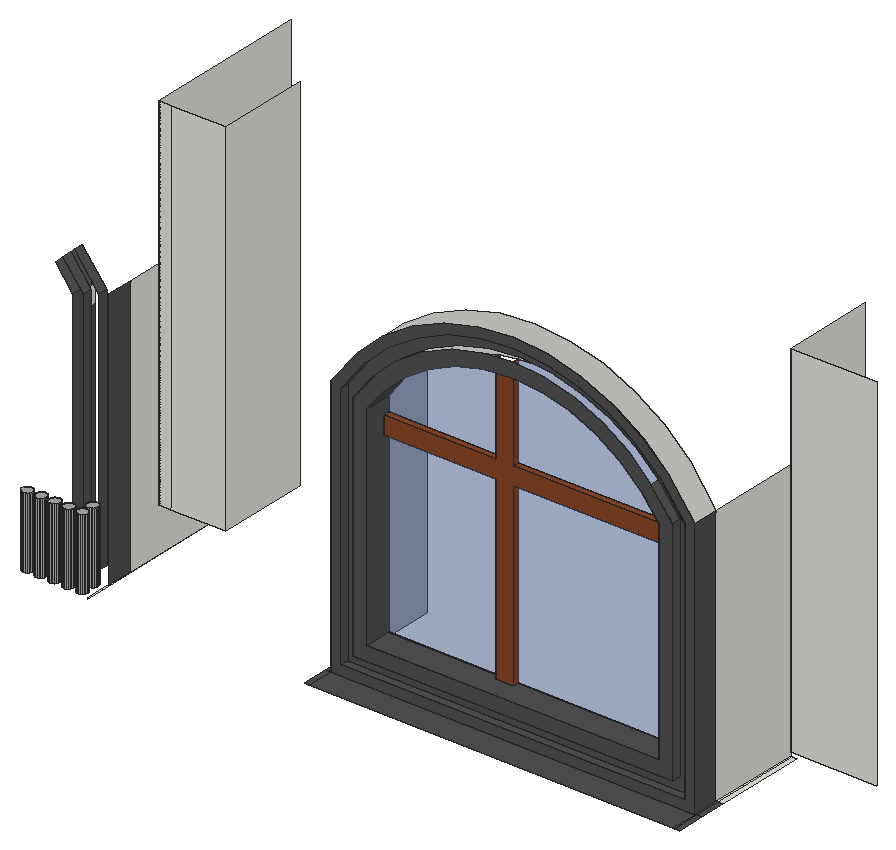
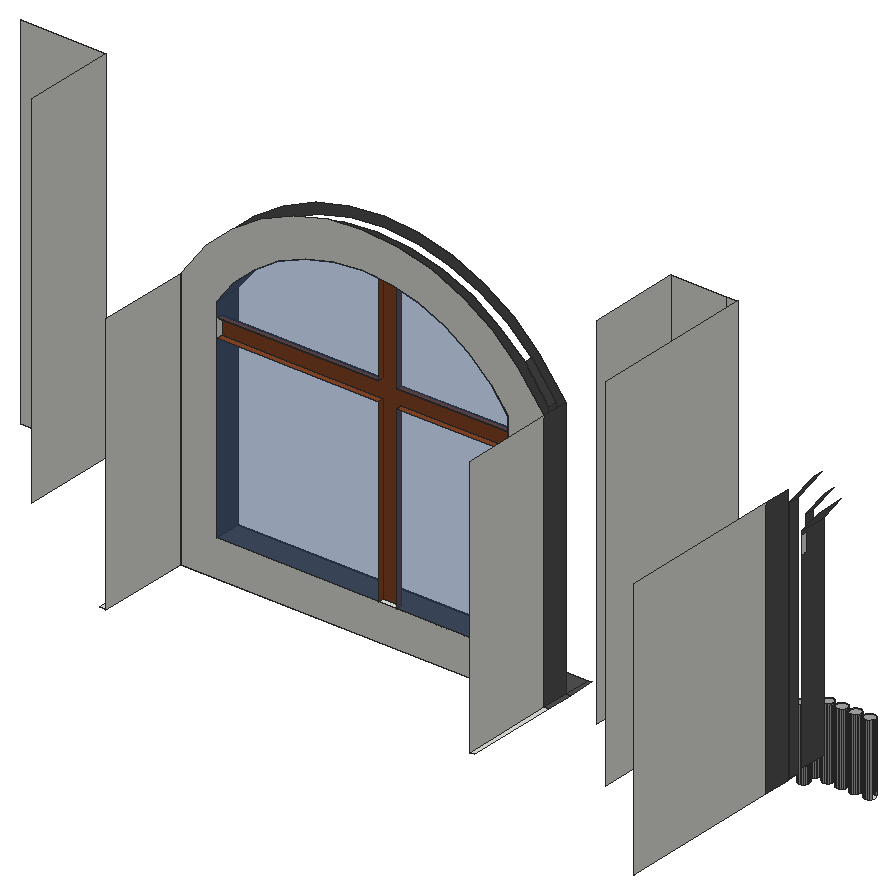
# SketchUp Ruby script. Lengths in inches.
U = 1.inch
M = Sketchup.active_model
def pt(a) = Geom::Point3d.new(a.map { |v| v * U })
def face(e, loops, mat)
  f = e.add_face(loops[0].map { |a| pt(a) })
  loops[1..].each { |l| e.add_face(l.map { |a| pt(a) }).erase! }
  f.material = f.back_material = mat if mat
  f
end
# faces: each face lists its corners as indices into pts; further lists are holes
def faces(e, pts, list, mat = nil) = list.each { |f| face(e, (f[0].is_a?(Array) ? f : [f]).map { |l| l.map { |i| pts[i] } }, mat) }
# xy, xz, yz: faces in a plane at the given z, y or x. An outline is a flat list of corners, or four numbers for a rectangle; further outlines are holes
def ring(l) = l.size == 4 ? [[l[0], l[1]], [l[2], l[1]], [l[2], l[3]], [l[0], l[3]]] : l.each_slice(2).to_a
def flat(e, list, mat, &to3) = list.each { |f| face(e, (f[0].is_a?(Array) ? f : [f]).map { |l| ring(l).map { |u, v| to3.(u, v) } }, mat) }
def xy(e, z, list, mat = nil) = flat(e, list, mat) { |x, y| [x, y, z] }
def xz(e, y, list, mat = nil) = flat(e, list, mat) { |x, z| [x, y, z] }
def yz(e, x, list, mat = nil) = flat(e, list, mat) { |y, z| [x, y, z] }
def lines(e, pts, list) = list.each { |a, b| e.add_line(pt(pts[a]), pt(pts[b])) }
# prism: a flat outline (further loops are holes) pulled along v
def prism(e, loops, v, mat = nil)
  f = face(e, loops, mat); d = Geom::Vector3d.new(v.map { |x| x * U })
  f.pushpull(f.normal.samedirection?(d) ? d.length : -d.length)
end
def box(e, o, s, mat = nil) = prism(e, [[o, [o[0] + s[0], o[1], o[2]], [o[0] + s[0], o[1] + s[1], o[2]], [o[0], o[1] + s[1], o[2]]]], [0, 0, s[2]], mat)
def at(x, y, z, deg = 0) = Geom::Transformation.translation(pt([x, y, z])) * Geom::Transformation.rotation(ORIGIN, Z_AXIS, deg.degrees)
def axes(o, x, y, z) = Geom::Transformation.new([*x, 0, *y, 0, *z, 0, *pt(o).to_a, 1])
def part(name) = M.definitions.add(name)
# library, detail: a bought-in or finely detailed component or shape, given as its bounding box
def library(name, o, s) = part(name).tap { |d| box(d.entities, o, s) }
def detail(e, o, s) = box(e.add_group.entities, o, s)
def put(e, d, t, mat = nil) = e.add_instance(d, t).tap { |i| i.material = mat if mat }
def group(e, t, mat = nil) = e.add_group.tap { |g| g.transformation = t; g.material = mat if mat }.entities
root = M.entities
M.materials.add("[0042_Sienna]").color = [137, 70, 38]
M.materials.add("[0132_LightGray]").color = [169, 169, 169]
M.materials.add("[0135_DarkGray]").color = [81, 81, 81]
M.materials.add("[Translucent Glass Blue]").color = [66, 99, 158]
M.materials["[Translucent Glass Blue]"].alpha = 0.5
xy(root,336.85,[[361.14,31.6875,361.32,37.6875],[339.27,32.1,338.81,32.2,338.39,32.42,338.04,32.73,337.78,33.13,337.63,33.58,337.61,34.05,337.7,34.52,337.92,34.9375,338.23,35.29,338.63,35.55,339.08,35.69,339.55,35.72,340.02,35.62,340.4375,35.41,340.79,35.09,341.05,34.69,341.19,34.24,341.22,33.77,341.12,33.31,340.91,32.89,340.59,32.53,340.19,32.28,339.74,32.13],[343.83,32.1,343.37,32.2,342.95,32.42,342.6,32.73,342.34,33.13,342.19,33.58,342.17,34.05,342.27,34.52,342.48,34.9375,342.8,35.29,343.19,35.55,343.64,35.69,344.12,35.72,344.58,35.62,345,35.41,345.35,35.09,345.61,34.69,345.76,34.24,345.78,33.77,345.68,33.31,345.47,32.89,345.15,32.53,344.76,32.28,344.31,32.13],[348.4,32.1,347.93,32.2,347.51,32.42,347.16,32.73,346.9,33.13,346.76,33.58,346.73,34.05,346.83,34.52,347.04,34.9375,347.36,35.29,347.76,35.55,348.21,35.69,348.68,35.72,349.14,35.62,349.5625,35.41,349.92,35.09,350.17,34.69,350.32,34.24,350.34,33.77,350.25,33.31,350.03,32.89,349.72,32.53,349.32,32.28,348.87,32.13],[352.96,32.1,352.5,32.2,352.07,32.42,351.72,32.73,351.47,33.13,351.32,33.58,351.29,34.05,351.39,34.52,351.61,34.9375,351.92,35.29,352.32,35.55,352.77,35.69,353.24,35.72,353.7,35.62,354.125,35.41,354.48,35.09,354.74,34.69,354.88,34.24,354.91,33.77,354.81,33.31,354.59,32.89,354.28,32.53,353.88,32.28,353.43,32.13],
  [357.52,32.1,357.06,32.2,356.64,32.42,356.29,32.73,356.03,33.13,355.88,33.58,355.86,34.05,355.95,34.52,356.17,34.9375,356.48,35.29,356.88,35.55,357.33,35.69,357.8,35.72,358.27,35.62,358.6875,35.41,359.04,35.09,359.3,34.69,359.44,34.24,359.47,33.77,359.37,33.31,359.16,32.89,358.84,32.53,358.44,32.28,357.99,32.13],[361.14,37.6875,361.32,49.6875],[434.7,40.6875,555.39,49.6875],[361.14,49.6875,361.32,104.375],[433.14,49.6875,434.7,80.4375],
  [555.39,49.6875,556.01,80.4375],[556.01,49.6875,557.64,80.4375]])
xy(root,336.85,[[433.14,31.6875,434.7,40.6875],[434.7,31.6875,555.39,40.6875],[555.39,31.6875,556.01,40.6875],[556.01,31.6875,557.64,40.6875],[433.14,40.6875,434.7,49.6875],
  [555.39,40.6875,556.01,49.6875],[556.01,40.6875,557.64,49.6875]],"[0135_DarkGray]")
xy(root,340.02,[[437.88,40.6875,552.21,43.6875]],"[0135_DarkGray]")
xy(root,344.17,[[442.02,40.6875,548.06,43.6875]],"[0135_DarkGray]")
xy(root,348.85,[[483.7,47.6875,489.7,49.6875]])
xy(root,348.85,[[446.7,40.6875,543.39,40.6875,543.39,49.6875,489.7,49.6875,489.7,47.6875,483.7,47.6875,483.7,49.6875,446.7,49.6875]],"[0135_DarkGray]")
xy(root,360.41,[[339.27,32.1,339.74,32.13,340.19,32.28,340.59,32.53,340.91,32.89,341.12,33.31,341.22,33.77,341.19,34.24,341.05,34.69,340.79,35.09,340.4375,35.41,340.02,35.62,339.55,35.72,339.08,35.69,338.63,35.55,338.23,35.29,337.92,34.9375,337.7,34.52,337.61,34.05,337.63,33.58,337.78,33.13,338.04,32.73,338.39,32.42,338.81,32.2],[343.83,32.1,344.31,32.13,344.76,32.28,345.15,32.53,345.47,32.89,345.68,33.31,345.78,33.77,345.76,34.24,345.61,34.69,345.35,35.09,345,35.41,344.58,35.62,344.12,35.72,343.64,35.69,343.19,35.55,342.8,35.29,342.48,34.9375,342.27,34.52,342.17,34.05,342.19,33.58,342.34,33.13,342.6,32.73,342.95,32.42,343.37,32.2],[348.4,32.1,348.87,32.13,349.32,32.28,349.72,32.53,350.03,32.89,350.25,33.31,350.34,33.77,350.32,34.24,350.17,34.69,349.92,35.09,349.5625,35.41,349.14,35.62,348.68,35.72,348.21,35.69,347.76,35.55,347.36,35.29,347.04,34.9375,346.83,34.52,346.73,34.05,346.76,33.58,346.9,33.13,347.16,32.73,347.51,32.42,347.93,32.2],[352.96,32.1,353.43,32.13,353.88,32.28,354.28,32.53,354.59,32.89,354.81,33.31,354.91,33.77,354.88,34.24,354.74,34.69,354.48,35.09,354.125,35.41,353.7,35.62,353.24,35.72,352.77,35.69,352.32,35.55,351.92,35.29,351.61,34.9375,351.39,34.52,351.29,34.05,351.32,33.58,351.47,33.13,351.72,32.73,352.07,32.42,352.5,32.2],[357.52,32.1,357.99,32.13,358.44,32.28,358.84,32.53,359.16,32.89,359.37,33.31,359.47,33.77,359.44,34.24,359.3,34.69,359.04,35.09,358.6875,35.41,358.27,35.62,357.8,35.72,357.33,35.69,356.88,35.55,356.48,35.29,356.17,34.9375,355.95,34.52,355.86,34.05,355.88,33.58,356.03,33.13,356.29,32.73,356.64,32.42,357.06,32.2],
  [357.52,36.54,357.99,36.57,358.44,36.71,358.84,36.97,359.16,37.32,359.37,37.75,359.47,38.21,359.44,38.68,359.3,39.13,359.04,39.53,358.6875,39.84,358.27,40.06,357.8,40.16,357.33,40.13,356.88,39.98,356.48,39.73,356.17,39.375,355.95,38.95,355.86,38.49,355.88,38.02,356.03,37.57,356.29,37.17,356.64,36.85,357.06,36.64]],"[0132_LightGray]")
xy(root,408.35,[[446.7,47.6875,483.7,49.6875],[489.7,47.6875,543.39,49.6875]],"[0042_Sienna]")
xy(root,414.35,[[446.7,47.6875,483.7,49.6875],[489.7,47.6875,543.39,49.6875]],"[0042_Sienna]")
xz(root,40.6875,[[[434.7,336.85,555.39,336.85,555.39,423.26,546.46,434.86,537.99,442.73,528.34,449.09,517.76,453.76,506.5625,456.61,495.04,457.57,483.52,456.61,472.32,453.76,461.75,449.09,452.09,442.73,443.625,434.86,434.7,423.26],[437.88,340.02,437.88,422.18,445.98,432.71,454.0625,440.22,463.27,446.29,473.36,450.74,484.05,453.47,495.04,454.38,506.03,453.47,516.72,450.74,526.81,446.29,536.02,440.22,544.1,432.71,552.21,422.18,552.21,340.02]],[[442.02,344.17,548.06,344.17,548.06,420.77,541.02,429.91,533.45,436.95,524.82,442.63,515.36,446.81,505.34,449.36,495.04,450.22,484.74,449.36,474.72,446.81,465.27,442.63,456.63,436.95,449.06,429.91,442.02,420.77],[446.7,348.85,446.7,419.18,452.53,426.75,459.53,433.26,467.51,438.52,476.25,442.38,485.52,444.74,495.04,445.53,504.57,444.74,513.83,442.38,522.57,438.52,530.55,433.26,537.56,426.75,543.39,419.18,543.39,348.85]]],"[0135_DarkGray]")
xz(root,43.6875,[[[437.88,340.02,552.21,340.02,552.21,422.18,544.1,432.71,536.02,440.22,526.81,446.29,516.72,450.74,506.03,453.47,495.04,454.38,484.05,453.47,473.36,450.74,463.27,446.29,454.0625,440.22,445.98,432.71,437.88,422.18],[442.02,344.17,442.02,420.77,449.06,429.91,456.63,436.95,465.27,442.63,474.72,446.81,484.74,449.36,495.04,450.22,505.34,449.36,515.36,446.81,524.82,442.63,533.45,436.95,541.02,429.91,548.06,420.77,548.06,344.17]]],"[0135_DarkGray]")
xz(root,47.6875,[[483.7,348.85,489.7,348.85,489.7,408.35,543.39,408.35,543.39,414.35,489.7,414.35,489.7,445.09,485.52,444.74,483.7,444.27,483.7,414.35,446.7,414.35,446.7,408.35,483.7,408.35]],"[0042_Sienna]")
xz(root,49.6875,[[[434.7,336.85,434.7,423.26,443.625,434.86,452.09,442.73,461.75,449.09,472.32,453.76,483.52,456.61,495.04,457.57,506.5625,456.61,517.76,453.76,528.34,449.09,537.99,442.73,546.46,434.86,555.39,423.26,555.39,336.85],[446.7,348.85,543.39,348.85,543.39,419.18,537.56,426.75,530.55,433.26,522.57,438.52,513.83,442.38,504.57,444.74,495.04,445.53,489.7,445.09,485.52,444.74,483.7,444.27,476.25,442.38,467.51,438.52,459.53,433.26,452.53,426.75,446.7,419.18]],[370.55,360,370.74,480],[370.74,360,374.55,480],[374.55,360,392.7,480],[580.01,360,608.5,480]])
xz(root,49.6875,[[446.7,348.85,483.7,408.35],[489.7,348.85,543.39,408.35],[446.7,414.35,483.7,414.35,483.7,444.27,476.25,442.38,467.51,438.52,459.53,433.26,452.53,426.75,446.7,419.18],[489.7,414.35,543.39,414.35,543.39,419.18,537.56,426.75,530.55,433.26,522.57,438.52,513.83,442.38,504.57,444.74,495.04,445.53,489.7,445.09]],"[Translucent Glass Blue]")
yz(root,349.14,[[47.6875,412.18,49.6875,418.18]])
yz(root,349.14,[[40.6875,348.85,40.6875,419.18,49.6875,419.18,49.6875,418.18,47.6875,418.18,47.6875,412.18,49.6875,412.18,49.6875,348.85]],"[0135_DarkGray]")
yz(root,352.68,[[40.6875,345.3,43.6875,420.38]],"[0135_DarkGray]")
yz(root,357.84,[[40.6875,340.14,43.6875,422.14]],"[0135_DarkGray]")
yz(root,361.14,[[49.6875,336.85,104.375,423.26]])
yz(root,361.14,[[40.6875,336.85,49.6875,423.26]],"[0135_DarkGray]")
yz(root,370.55,[[49.6875,360,104.375,480]])
yz(root,392.7,[[49.6875,360,80.4375,480]])
yz(root,434.7,[[49.6875,336.85,80.4375,423.26]])
yz(root,434.7,[[40.6875,336.85,49.6875,423.26]],"[0135_DarkGray]")
yz(root,437.88,[[40.6875,340.02,43.6875,422.18]],"[0135_DarkGray]")
yz(root,442.02,[[40.6875,344.17,43.6875,420.77]],"[0135_DarkGray]")
yz(root,446.7,[[47.6875,408.35,49.6875,414.35]])
yz(root,446.7,[[40.6875,348.85,49.6875,348.85,49.6875,408.35,47.6875,408.35,47.6875,414.35,49.6875,414.35,49.6875,419.18,40.6875,419.18]],"[0135_DarkGray]")
yz(root,483.7,[[47.6875,348.85,49.6875,408.35],[47.6875,414.35,49.6875,444.27]],"[0042_Sienna]")
yz(root,489.7,[[47.6875,348.85,49.6875,408.35],[47.6875,414.35,49.6875,445.09]],"[0042_Sienna]")
yz(root,543.39,[[47.6875,408.35,49.6875,414.35]])
yz(root,543.39,[[40.6875,348.85,40.6875,419.18,49.6875,419.18,49.6875,414.35,47.6875,414.35,47.6875,408.35,49.6875,408.35,49.6875,348.85]],"[0135_DarkGray]")
yz(root,548.06,[[40.6875,344.17,43.6875,420.77]],"[0135_DarkGray]")
yz(root,552.21,[[40.6875,340.02,43.6875,422.18]],"[0135_DarkGray]")
yz(root,555.39,[[49.6875,336.85,80.4375,423.26]])
yz(root,555.39,[[40.6875,336.85,49.6875,423.26]],"[0135_DarkGray]")
yz(root,580.01,[[49.6875,360,80.4375,480]])
p = [[338.81,32.2,336.85],[339.27,32.1,336.85],[339.27,32.1,360.41],[338.81,32.2,360.41],[339.74,32.13,336.85],[339.74,32.13,360.41],
  [340.19,32.28,336.85],[340.19,32.28,360.41],[343.37,32.2,336.85],[343.83,32.1,336.85],[343.83,32.1,360.41],[343.37,32.2,360.41],
  [344.31,32.13,336.85],[344.31,32.13,360.41],[344.76,32.28,336.85],[344.76,32.28,360.41],[347.93,32.2,336.85],[348.4,32.1,336.85],
  [348.4,32.1,360.41],[347.93,32.2,360.41],[348.87,32.13,336.85],[348.87,32.13,360.41],[349.32,32.28,336.85],[349.32,32.28,360.41],
  [352.5,32.2,336.85],[352.96,32.1,336.85],[352.96,32.1,360.41],[352.5,32.2,360.41],[353.43,32.13,336.85],[353.43,32.13,360.41],
  [353.88,32.28,336.85],[353.88,32.28,360.41],[357.06,32.2,336.85],[357.52,32.1,336.85],[357.52,32.1,360.41],[357.06,32.2,360.41],
  [357.99,32.13,336.85],[357.99,32.13,360.41],[358.44,32.28,336.85],[358.44,32.28,360.41],[338.39,32.42,336.85],[338.39,32.42,360.41],
  [342.95,32.42,336.85],[342.95,32.42,360.41],[347.51,32.42,336.85],[347.51,32.42,360.41],[352.07,32.42,336.85],[352.07,32.42,360.41],
  [356.64,32.42,336.85],[356.64,32.42,360.41],[340.59,32.53,336.85],[340.59,32.53,360.41],[345.15,32.53,336.85],[345.15,32.53,360.41],
  [349.72,32.53,336.85],[349.72,32.53,360.41],[354.28,32.53,336.85],[354.28,32.53,360.41],[358.84,32.53,336.85],[358.84,32.53,360.41],
  [338.04,32.73,336.85],[338.04,32.73,360.41],[342.6,32.73,336.85],[342.6,32.73,360.41],[347.16,32.73,336.85],[347.16,32.73,360.41],
  [351.72,32.73,336.85],[351.72,32.73,360.41],[356.29,32.73,336.85],[356.29,32.73,360.41],[340.91,32.89,336.85],[340.91,32.89,360.41],
  [345.47,32.89,336.85],[345.47,32.89,360.41],[350.03,32.89,336.85],[350.03,32.89,360.41],[354.59,32.89,336.85],[354.59,32.89,360.41],
  [359.16,32.89,336.85],[359.16,32.89,360.41],[342.34,33.13,336.85],[342.34,33.13,360.41],[346.9,33.13,336.85],[346.9,33.13,360.41],
  [351.47,33.13,336.85],[351.47,33.13,360.41],[356.03,33.13,336.85],[356.03,33.13,360.41],[341.12,33.31,336.85],[341.12,33.31,360.41],
  [345.68,33.31,336.85],[345.68,33.31,360.41],[350.25,33.31,336.85],[350.25,33.31,360.41],[354.81,33.31,336.85],[354.81,33.31,360.41],
  [359.37,33.31,336.85],[359.37,33.31,360.41],[342.19,33.58,336.85],[342.19,33.58,360.41],[346.76,33.58,336.85],[346.76,33.58,360.41],
  [351.32,33.58,336.85],[351.32,33.58,360.41],[355.88,33.58,336.85],[355.88,33.58,360.41],[341.22,33.77,336.85],[341.22,33.77,360.41],
  [345.78,33.77,336.85],[345.78,33.77,360.41],[350.34,33.77,336.85],[350.34,33.77,360.41],[354.91,33.77,336.85],[354.91,33.77,360.41],
  [359.47,33.77,336.85],[359.47,33.77,360.41],[342.17,34.05,336.85],[342.17,34.05,360.41],[346.73,34.05,336.85],[346.73,34.05,360.41],
  [351.29,34.05,336.85],[351.29,34.05,360.41],[355.86,34.05,336.85],[355.86,34.05,360.41],[341.19,34.24,336.85],[341.19,34.24,360.41],
  [345.76,34.24,336.85],[345.76,34.24,360.41],[350.32,34.24,336.85],[350.32,34.24,360.41],[354.88,34.24,336.85],[354.88,34.24,360.41],
  [359.44,34.24,336.85],[359.44,34.24,360.41],[342.27,34.52,336.85],[342.27,34.52,360.41],[346.83,34.52,336.85],[346.83,34.52,360.41],
  [351.39,34.52,336.85],[351.39,34.52,360.41],[355.95,34.52,336.85],[355.95,34.52,360.41],[341.05,34.69,336.85],[341.05,34.69,360.41],
  [345.61,34.69,336.85],[345.61,34.69,360.41],[350.17,34.69,336.85],[350.17,34.69,360.41],[354.74,34.69,336.85],[354.74,34.69,360.41],
  [359.3,34.69,336.85],[359.3,34.69,360.41],[342.48,34.9375,336.85],[342.48,34.9375,360.41],[347.04,34.9375,336.85],[347.04,34.9375,360.41],
  [351.61,34.9375,336.85],[351.61,34.9375,360.41],[356.17,34.9375,336.85],[356.17,34.9375,360.41],[340.79,35.09,336.85],[340.79,35.09,360.41],
  [345.35,35.09,336.85],[345.35,35.09,360.41],[349.92,35.09,336.85],[349.92,35.09,360.41],[354.48,35.09,336.85],[354.48,35.09,360.41],
  [359.04,35.09,336.85],[359.04,35.09,360.41],[338.23,35.29,336.85],[337.92,34.9375,336.85],[337.92,34.9375,360.41],[338.23,35.29,360.41],
  [342.8,35.29,336.85],[342.8,35.29,360.41],[347.36,35.29,336.85],[347.36,35.29,360.41],[351.92,35.29,336.85],[351.92,35.29,360.41],
  [356.48,35.29,336.85],[356.48,35.29,360.41],[340.4375,35.41,336.85],[340.4375,35.41,360.41],[345,35.41,336.85],[345,35.41,360.41],
  [349.5625,35.41,336.85],[349.5625,35.41,360.41],[354.125,35.41,336.85],[354.125,35.41,360.41],[358.6875,35.41,336.85],[358.6875,35.41,360.41],
  [338.63,35.55,336.85],[338.63,35.55,360.41],[343.19,35.55,336.85],[343.19,35.55,360.41],[347.76,35.55,336.85],[347.76,35.55,360.41],
  [352.32,35.55,336.85],[352.32,35.55,360.41],[356.88,35.55,336.85],[356.88,35.55,360.41],[340.02,35.62,336.85],[340.02,35.62,360.41],
  [344.58,35.62,336.85],[344.58,35.62,360.41],[349.14,35.62,336.85],[349.14,35.62,360.41],[353.7,35.62,336.85],[353.7,35.62,360.41],
  [358.27,35.62,336.85],[358.27,35.62,360.41],[339.08,35.69,336.85],[339.08,35.69,360.41],[343.64,35.69,336.85],[343.64,35.69,360.41],
  [348.21,35.69,336.85],[348.21,35.69,360.41],[352.77,35.69,336.85],[352.77,35.69,360.41],[357.33,35.69,336.85],[357.33,35.69,360.41],
  [339.55,35.72,336.85],[339.55,35.72,360.41],[344.12,35.72,336.85],[344.12,35.72,360.41],[348.68,35.72,336.85],[348.68,35.72,360.41],
  [353.24,35.72,336.85],[353.24,35.72,360.41],[357.8,35.72,336.85],[357.8,35.72,360.41],[357.06,36.64,336.85],[357.52,36.54,336.85],
  [357.52,36.54,360.41],[357.06,36.64,360.41],[357.99,36.57,336.85],[357.99,36.57,360.41],[356.64,36.85,336.85],[356.64,36.85,360.41],
  [358.44,36.71,336.85],[358.44,36.71,360.41],[358.84,36.97,336.85],[358.84,36.97,360.41],[356.29,37.17,336.85],[356.29,37.17,360.41],
  [359.16,37.32,336.85],[359.16,37.32,360.41],[356.03,37.57,336.85],[356.03,37.57,360.41],[359.37,37.75,336.85],[359.37,37.75,360.41],
  [355.88,38.02,336.85],[355.88,38.02,360.41],[359.47,38.21,336.85],[359.47,38.21,360.41],[355.86,38.49,336.85],[355.86,38.49,360.41],
  [359.44,38.68,336.85],[359.44,38.68,360.41],[355.95,38.95,336.85],[355.95,38.95,360.41],[359.3,39.13,336.85],[359.3,39.13,360.41],
  [356.17,39.375,336.85],[356.17,39.375,360.41],[359.04,39.53,336.85],[359.04,39.53,360.41],[356.48,39.73,336.85],[356.48,39.73,360.41],
  [358.6875,39.84,336.85],[358.6875,39.84,360.41],[356.88,39.98,336.85],[356.88,39.98,360.41],[358.27,40.06,336.85],[358.27,40.06,360.41],
  [357.33,40.13,336.85],[357.33,40.13,360.41],[357.8,40.16,336.85],[357.8,40.16,360.41],[343.31,49.6875,426.75],[349.14,49.6875,419.18],
  [349.14,40.6875,419.18],[343.31,40.6875,426.75],[446.7,49.6875,419.18],[452.53,49.6875,426.75],[452.53,40.6875,426.75],[446.7,40.6875,419.18],
  [537.56,49.6875,426.75],[543.39,49.6875,419.18],[543.39,40.6875,419.18],[537.56,40.6875,426.75],[352.68,43.6875,420.38],[345.9375,43.6875,429.15],
  [345.9375,40.6875,429.15],[352.68,40.6875,420.38],[449.06,43.6875,429.91],[442.02,43.6875,420.77],[442.02,40.6875,420.77],[449.06,40.6875,429.91],
  [548.06,43.6875,420.77],[541.02,43.6875,429.91],[541.02,40.6875,429.91],[548.06,40.6875,420.77],[349.77,43.6875,432.64],[357.84,43.6875,422.14],
  [357.84,40.6875,422.14],[349.77,40.6875,432.64],[437.88,43.6875,422.18],[445.98,43.6875,432.71],[445.98,40.6875,432.71],[437.88,40.6875,422.18],
  [544.1,43.6875,432.71],[552.21,43.6875,422.18],[552.21,40.6875,422.18],[544.1,40.6875,432.71]]
faces(root,p,[[0,1,2,3],[1,4,5,2],[4,6,7,5],[8,9,10,11],[9,12,13,10],[12,14,15,13],[16,17,18,19],[17,20,21,18],
  [20,22,23,21],[24,25,26,27],[25,28,29,26],[28,30,31,29],[32,33,34,35],[33,36,37,34],[36,38,39,37],[40,0,3,41],
  [42,8,11,43],[44,16,19,45],[46,24,27,47],[48,32,35,49],[6,50,51,7],[14,52,53,15],[22,54,55,23],[30,56,57,31],
  [38,58,59,39],[60,40,41,61],[62,42,43,63],[64,44,45,65],[66,46,47,67],[68,48,49,69],[50,70,71,51],[52,72,73,53],
  [54,74,75,55],[56,76,77,57],[58,78,79,59],[80,62,63,81],[82,64,65,83],[84,66,67,85],[86,68,69,87],[70,88,89,71],
  [72,90,91,73],[74,92,93,75],[76,94,95,77],[78,96,97,79],[98,80,81,99],[100,82,83,101],[102,84,85,103],[104,86,87,105],
  [88,106,107,89],[90,108,109,91],[92,110,111,93],[94,112,113,95],[96,114,115,97],[116,98,99,117],[118,100,101,119],[120,102,103,121],
  [122,104,105,123],[106,124,125,107],[108,126,127,109],[110,128,129,111],[112,130,131,113],[114,132,133,115],[134,116,117,135],[136,118,119,137],
  [138,120,121,139],[140,122,123,141],[124,142,143,125],[126,144,145,127],[128,146,147,129],[130,148,149,131],[132,150,151,133],[152,134,135,153],
  [154,136,137,155],[156,138,139,157],[158,140,141,159],[142,160,161,143],[144,162,163,145],[146,164,165,147],[148,166,167,149],[150,168,169,151],
  [170,171,172,173],[174,152,153,175],[176,154,155,177],[178,156,157,179],[180,158,159,181],[160,182,183,161],[162,184,185,163],[164,186,187,165],
  [166,188,189,167],[168,190,191,169],[192,170,173,193],[194,174,175,195],[196,176,177,197],[198,178,179,199],[200,180,181,201],[182,202,203,183],
  [184,204,205,185],[186,206,207,187],[188,208,209,189],[190,210,211,191],[212,192,193,213],[214,194,195,215],[216,196,197,217],[218,198,199,219],
  [220,200,201,221],[202,222,223,203],[204,224,225,205],[206,226,227,207],[208,228,229,209],[210,230,231,211],[222,212,213,223],[224,214,215,225],
  [226,216,217,227],[228,218,219,229],[230,220,221,231],[232,233,234,235],[233,236,237,234],[238,232,235,239],[236,240,241,237],[240,242,243,241],
  [244,238,239,245],[242,246,247,243],[248,244,245,249],[246,250,251,247],[252,248,249,253],[250,254,255,251],[256,252,253,257],[254,258,259,255],
  [260,256,257,261],[258,262,263,259],[264,260,261,265],[262,266,267,263],[268,264,265,269],[266,270,271,267],[272,268,269,273],[270,274,275,271],
  [276,272,273,277],[278,276,277,279],[274,278,279,275]],"[0132_LightGray]")
faces(root,p,[[280,281,282,283],[284,285,286,287],[288,289,290,291],[292,293,294,295],[296,297,298,299],[300,301,302,303],[304,305,306,307],[308,309,310,311],
  [312,313,314,315]],"[0135_DarkGray]")
